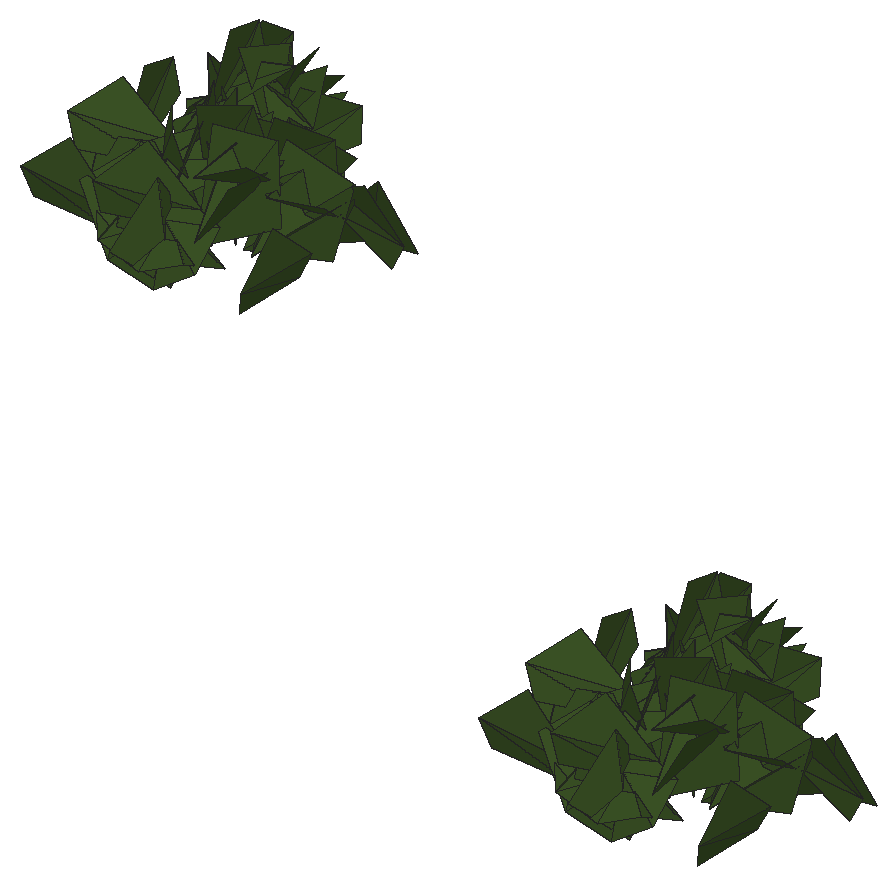
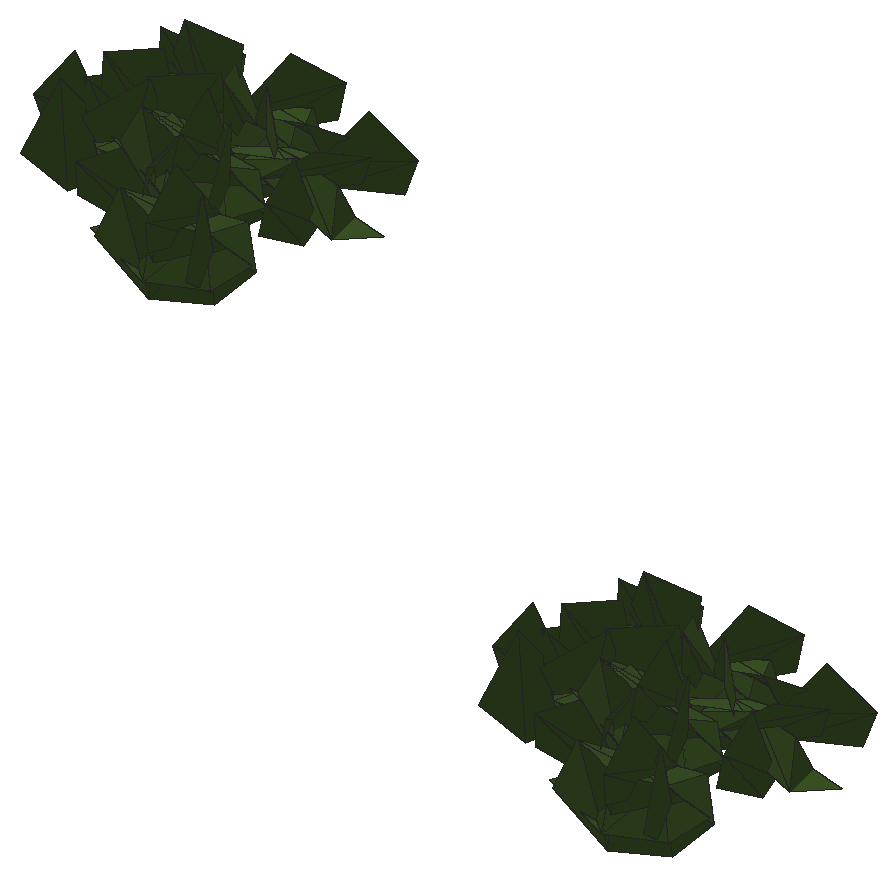
# SketchUp Ruby script. Lengths in inches.
U = 1.inch
M = Sketchup.active_model
def pt(a) = Geom::Point3d.new(a.map { |v| v * U })
def face(e, loops, mat)
  f = e.add_face(loops[0].map { |a| pt(a) })
  loops[1..].each { |l| e.add_face(l.map { |a| pt(a) }).erase! }
  f.material = f.back_material = mat if mat
  f
end
# faces: each face lists its corners as indices into pts; further lists are holes
def faces(e, pts, list, mat = nil) = list.each { |f| face(e, (f[0].is_a?(Array) ? f : [f]).map { |l| l.map { |i| pts[i] } }, mat) }
# xy, xz, yz: faces in a plane at the given z, y or x. An outline is a flat list of corners, or four numbers for a rectangle; further outlines are holes
def ring(l) = l.size == 4 ? [[l[0], l[1]], [l[2], l[1]], [l[2], l[3]], [l[0], l[3]]] : l.each_slice(2).to_a
def flat(e, list, mat, &to3) = list.each { |f| face(e, (f[0].is_a?(Array) ? f : [f]).map { |l| ring(l).map { |u, v| to3.(u, v) } }, mat) }
def xy(e, z, list, mat = nil) = flat(e, list, mat) { |x, y| [x, y, z] }
def xz(e, y, list, mat = nil) = flat(e, list, mat) { |x, z| [x, y, z] }
def yz(e, x, list, mat = nil) = flat(e, list, mat) { |y, z| [x, y, z] }
def lines(e, pts, list) = list.each { |a, b| e.add_line(pt(pts[a]), pt(pts[b])) }
# prism: a flat outline (further loops are holes) pulled along v
def prism(e, loops, v, mat = nil)
  f = face(e, loops, mat); d = Geom::Vector3d.new(v.map { |x| x * U })
  f.pushpull(f.normal.samedirection?(d) ? d.length : -d.length)
end
def box(e, o, s, mat = nil) = prism(e, [[o, [o[0] + s[0], o[1], o[2]], [o[0] + s[0], o[1] + s[1], o[2]], [o[0], o[1] + s[1], o[2]]]], [0, 0, s[2]], mat)
def at(x, y, z, deg = 0) = Geom::Transformation.translation(pt([x, y, z])) * Geom::Transformation.rotation(ORIGIN, Z_AXIS, deg.degrees)
def axes(o, x, y, z) = Geom::Transformation.new([*x, 0, *y, 0, *z, 0, *pt(o).to_a, 1])
def part(name) = M.definitions.add(name)
# library, detail: a bought-in or finely detailed component or shape, given as its bounding box
def library(name, o, s) = part(name).tap { |d| box(d.entities, o, s) }
def detail(e, o, s) = box(e.add_group.entities, o, s)
def put(e, d, t, mat = nil) = e.add_instance(d, t).tap { |i| i.material = mat if mat }
def group(e, t, mat = nil) = e.add_group.tap { |g| g.transformation = t; g.material = mat if mat }.entities
root = M.entities
M.materials.add("AM113_062_Tilia").color = [58, 81, 37]
p = [[1505.11,269.32,879.56],[1479.46,218.66,800.37],[1525.74,267.35,750.21],[1495.65,353.01,772.9],[344.49,918.09,879.56],[318.83,867.43,800.37],
  [365.11,916.125,750.21],[335.03,1001.78,772.9],[1444.78,257.76,760.62],[1516.15,249.39,752.03],[1512.28,272.93,827.79],[1563.2,262.4375,781.5],
  [284.15,906.53,760.62],[355.52,898.16,752.03],[351.66,921.7,827.79],[402.58,911.21,781.5],[1469.94,338.33,894.66],[1416.86,370.14,789.43],
  [1504.72,364.1,753.02],[309.3125,987.1,894.66],[256.24,1018.91,789.43],[344.09,1012.88,753.02],[1461.97,351.04,837.04],[1403.56,330.78,827.9],
  [1440.77,321.16,753.15],[1558.1,408.4,788.02],[301.35,999.8125,837.04],[242.93,979.56,827.9],[280.14,969.9375,753.15],[397.47,1057.18,788.02],
  [1384.37,557.68,884.94],[1368.75,544.08,755.59],[1451.59,506.93,778.28],[1365.28,611.16,805.75],[223.74,1206.46,884.94],[208.12,1192.85,755.59],
  [290.96,1155.71,778.28],[204.66,1259.9375,805.75],[1362.32,563.4,757.41],[1339.39,520.28,786.88],[1382.05,550,833.17],[1417.52,609.4,766],
  [201.69,1212.17,757.41],[178.76,1169.06,786.88],[221.43,1198.77,833.17],[256.89,1258.18,766],[1495.8,362.42,894.91],[1528.69,376.13,757.66],
  [1472.84,447.97,903.28],[1472.14,451.88,794.27],[335.17,1011.2,894.91],[368.07,1024.91,757.66],[312.22,1096.75,903.28],[311.52,1100.65,794.27],
  [1422.23,330.12,860.63],[1387.5,281.1,830.54],[1455.6,274.96,844.76],[261.61,978.89,860.63],[226.875,929.875,830.54],[294.97,923.73,844.76],
  [1685.92,428.47,868.25],[1643,469.68,760.75],[1601.23,388.02,775.93],[1718.77,458.36,776.85],[525.29,1077.24,868.25],[482.38,1118.45,760.75],
  [440.6,1036.8,775.93],[558.14,1107.14,776.85],[1558.49,353.8,770.9],[1643.65,403.42,764.22],[1669.83,408.41,867.79],[397.86,1002.58,770.9],
  [483.02,1052.19,764.22],[509.21,1057.1875,867.79],[1651.39,231.9,800.74],[1637.08,248.37,765.32],[1643.84,342.85,771.39],[490.77,880.68,800.74],
  [476.45,897.14,765.32],[483.21,991.625,771.39],[1510.12,285.74,822.95],[1557.17,250.19,797.3],[1562.42,315.02,765.59],[1425.7,366.6875,800.79],
  [349.49,934.51,822.95],[396.55,898.97,797.3],[401.8,963.8,765.59],[265.08,1015.46,800.79],[1422.54,589.72,850.14],[1485.52,575.95,866.01],
  [1473.88,634.88,835.92],[261.92,1238.49,850.14],[324.9,1224.72,866.01],[313.25,1283.66,835.92],[1353.5625,328.99,768.02],[1421.73,326.25,798.38],
  [1398.51,372.99,844.8],[1309.58,425.48,797.16],[1282.33,367.79,785.46],[1341.2,374.58,831.69],[192.9375,977.77,768.02],[261.1,975.03,798.38],
  [237.88,1021.76,844.8],[148.95,1074.26,797.16],[121.7,1016.57,785.46],[180.57,1023.35,831.69],[1565.52,422.83,908.3],[1570.57,466.93,789.28],
  [1547.93,378.67,768.94],[404.89,1071.6,908.3],[409.95,1115.71,789.28],[387.3,1027.45,768.94],[1585.97,394.56,901.01],[425.35,1043.33,901.01],
  [1413.57,298.3,770.99],[1430.23,294.69,796.45],[1312.58,269.91,826.9],[1320.73,282.97,786.25],[1392.83,542.75,828.34],[1334.66,533.09,802.68],
  [1378.07,484.65,770.97],[1509.66,548.26,806.17],[252.95,947.08,770.99],[269.6,943.47,796.45],[151.95,918.68,826.9],[160.1,931.75,786.25],
  [232.21,1191.52,828.34],[174.03,1181.86,802.68],[217.44,1133.42,770.97],[349.04,1197.03,806.17],[1487.9,508.69,771.26],[1468.25,501.02,791.03],
  [1561.72,556.84,863.53],[1564.38,550.76,819.11],[327.27,1157.47,771.26],[307.62,1149.79,791.03],[401.1,1205.62,863.53],[403.76,1199.53,819.11],
  [1653.78,354.39,798.69],[493.15,1003.17,798.69],[1350.65,421.7,773.0625],[1347.38,400.18,791.58],[1336.71,506.75,868.36],[1345.75,507.56,824.65],
  [190.03,1070.48,773.0625],[186.75,1048.96,791.58],[176.08,1155.53,868.36],[185.125,1156.34,824.65],[1501.6,378.68,917.83],[1544.36,423.41,812.6],
  [1519.05,339.0625,776.1875],[340.97,1027.45,917.83],[383.74,1072.1875,812.6],[358.43,987.84,776.1875],[1515.76,383.64,860.21],[1491.3125,410.92,776.32],
  [1550.46,277.21,811.19],[1508.92,445.09,851.07],[355.13,1032.41,860.21],[330.6875,1059.7,776.32],[389.83,925.99,811.19],[348.29,1093.86,851.07],
  [1437.12,249.91,786.11],[1509.2,232.2,779.4],[276.49,898.6875,786.11],[348.57,880.97,779.4],[1562.21,426.5625,847.86],[1513.07,446.8,780.26],
  [1594.53,322.58,788.5],[1545.51,486.28,841.09],[401.58,1075.34,847.86],[352.44,1095.58,780.26],[433.9,971.36,788.5],[384.88,1135.06,841.09],
  [1519.38,348.13,918.08],[1525.49,313.02,780.83],[1607.89,351.61,926.45],[1611.86,351.43,817.4375],[358.76,996.91,918.08],[364.86,961.8,780.83],
  [447.26,1000.38,926.45],[451.23,1000.2,817.4375],[1561.01,307.91,820.32],[400.38,956.69,820.32],[1743.47,403,818.28],[1723.06,407.125,781.875],
  [1632.79,427.18,809.1],[582.85,1051.77,818.28],[562.43,1055.9,781.875],[472.17,1075.95,809.1],[1354.63,580.28,784.78],[1417.1,620.36,791.49],
  [194.01,1229.05,784.78],[256.47,1269.13,791.49],[1432.96,463.53,862.68],[1378.53,452.98,826.2],[1430.25,418.54,785.93],[1548.78,487.1,860.66],
  [272.33,1112.3,862.68],[217.91,1101.76,826.2],[269.62,1067.32,785.93],[388.16,1135.88,860.66],[1387.74,308.3,825.5625],[1456.53,303.2,834.19],
  [227.11,957.08,825.5625],[295.9,951.98,834.19],[1373.89,490.57,825.7],[213.26,1139.35,825.7],[1504.99,386.93,850.82],[1457.88,435.22,860.24],
  [1539.46,446.22,863.7],[344.37,1035.7,850.82],[297.25,1084,860.24],[378.83,1094.99,863.7],[1595.99,380.64,850.07],[1652.01,340.6,839.9375],
  [1647.35,422.57,831.44],[435.36,1029.41,850.07],[491.38,989.38,839.9375],[486.73,1071.35,831.44],[1625.83,466.75,859.6],[465.21,1115.53,859.6],
  [1417.88,402.8,880.25],[257.25,1051.58,880.25],[1418.98,464.77,920.71],[1413.49,477.46,789.83],[1499.13,446.82,811.375],[1397.37,530.43,860],
  [258.35,1113.54,920.71],[252.86,1126.23,789.83],[338.5,1095.6,811.375],[236.75,1179.2,860],[1509.96,513.43,887.34],[349.33,1162.2,887.34],
  [1442.39,569.6,839.57],[1493.45,615.98,830.94],[281.77,1218.375,839.57],[332.82,1264.76,830.94],[1350.2,440.18,890.34],[189.57,1088.95,890.34],
  [1369.71,285.49,875.14],[209.08,934.27,875.14],[1404.27,494.76,797.14],[1386.01,444.67,807.44],[1420.98,468.16,868.16],[1451.6,543.28,829.08],
  [243.64,1143.54,797.14],[225.38,1093.45,807.44],[260.36,1116.94,868.16],[290.98,1192.06,829.08],[1448.34,406.71,840.37],[287.71,1055.48,840.37],
  [1458.1,353.11,836.26],[297.48,1001.88,836.26],[1654.98,283.26,861.98],[494.35,932.04,861.98],[1641.14,426.9,803.98],[1587.47,475.04,799.73],
  [1566.1875,436.48,858.54],[1536.8,483.98,820.48],[480.51,1075.68,803.98],[426.84,1123.81,799.73],[405.5625,1085.26,858.54],[376.17,1132.76,820.48],
  [1452.61,350.8,849.62],[1404.99,328.4375,804.51],[1453.57,303.7,801.14],[1550.84,398.52,862.69],[291.98,999.58,849.62],[244.36,977.21,804.51],
  [292.9375,952.48,801.14],[390.21,1047.29,862.69],[1516.07,306.08,803.74],[1530.72,314.36,829.44],[1438.53,238.91,866.41],[1441.8125,249.07,823.32],
  [355.45,954.85,803.74],[370.1,963.13,829.44],[277.9,887.6875,866.41],[281.18,897.85,823.32],[1522.33,454.83,826.1],[1485.1,544.58,803.8],
  [1452.22,568.22,899.62],[361.7,1103.6,826.1],[324.48,1193.36,803.8],[291.59,1217,899.62],[1606.37,334.47,861.7],[1665.35,360.27,857.73],
  [1609.52,399.375,873.5625],[445.74,983.24,861.7],[504.72,1009.04,857.73],[448.89,1048.15,873.5625],[1408.25,382.2,807.54],[247.625,1030.98,807.54],
  [1468.59,347.9,804.99],[1476.13,323.85,813.625],[1474.53,406.84,929.89],[1466.92,417.58,887.95],[307.96,996.67,804.99],[315.5,972.625,813.625],
  [313.91,1055.62,929.89],[306.29,1066.36,887.95],[1316.74,348.23,862.76],[1332.6,342.68,823.04],[1411.1,394.51,807.43],[1418.08,412.34,830.27],
  [1421.9,412.07,839.76],[156.11,997.01,862.76],[171.97,991.46,823.04],[250.47,1043.28,807.43],[257.45,1061.11,830.27],[261.27,1060.85,839.76],
  [1452.02,436.32,832.12],[291.4,1085.1,832.12],[1624.69,427.32,841.08],[1403.49,524.43,809.125],[1399.41,508.1,834.82],[1408.15,626.91,871.79],
  [1413.26,617.54,828.7],[464.0625,1076.09,841.08],[242.86,1173.2,809.125],[238.78,1156.88,834.82],[247.52,1275.6875,871.79],[252.63,1266.31,828.7],
  [1541.25,333.75,873.99],[1598.77,369.02,883.4],[1591.45,287.03,886.87],[380.625,982.52,873.99],[438.14,1017.8,883.4],[430.83,935.8,886.87],
  [1575.99,415.2,903.42],[415.37,1063.97,903.42],[1506.07,345.47,914.42],[345.44,994.25,914.42],[1696.3,391.8125,883.47],[535.67,1040.59,883.47],
  [1549.97,418.79,820.17],[1529.32,414.35,839.91],[1638.67,412.5,911.18],[1637.79,416.86,866.3],[389.34,1067.57,820.17],[368.69,1063.125,839.91],
  [478.04,1061.28,911.18],[477.16,1065.64,866.3],[1508.93,438.33,834.43],[348.3,1087.1,834.43],[1517.6,392.82,872.79],[1471.45,402.3,824.31],
  [1542.42,286.48,885.86],[1506.32,444.21,827.68],[356.97,1041.6,872.79],[310.83,1051.08,824.31],[381.79,935.25,885.86],[345.69,1092.98,827.68],
  [1448.78,482.53,929.4],[288.16,1131.31,929.4],[1392.58,504.16,827.92],[231.96,1152.9375,827.92],[1558.03,429.14,830.7],[397.4,1077.92,830.7],
  [1407.17,382.28,843.86],[1448.05,548.27,857.14],[246.55,1031.05,843.86],[287.42,1197.05,857.14],[1511.24,377.88,828.15],[1486.12,375.84,836.79],
  [1567.41,359.05,953.05],[1579.56,364.1,911.12],[350.61,1026.66,828.15],[325.49,1024.62,836.79],[406.78,1007.83,953.05],[418.9375,1012.88,911.12],
  [1454.19,507.19,903.82],[1517.32,498,923.76],[1499.24,559.3,913.04],[293.57,1155.97,903.82],[356.69,1146.78,923.76],[338.62,1208.08,913.04],
  [1477.625,286.375,909.65],[317,935.15,909.65],[1344.25,409.57,888.11],[183.625,1058.34,888.11],[1601.13,374.49,855.29],[440.51,1023.27,855.29],
  [1597.59,477.85,833.46],[436.96,1126.63,833.46],[1487.08,391.2,880.42],[1520.22,451.73,887.98],[326.45,1039.98,880.42],[359.59,1100.51,887.98],
  [1415.66,565.88,915.03],[255.04,1214.65,915.03],[1500.58,341.87,937.59],[339.96,990.64,937.59],[1447.28,451.36,839.68],[1444,429.84,858.2],
  [1433.33,536.41,934.97],[1442.375,537.22,891.27],[286.65,1100.14,839.68],[283.375,1078.62,858.2],[272.71,1185.19,934.97],[281.75,1186,891.27],
  [1574.7,387.16,928.06],[414.08,1035.9375,928.06],[1558.34,430.18,867.03],[397.72,1078.95,867.03],[1601.09,304.58,911.14],[1549.38,350.28,903.59],
  [440.46,953.35,911.14],[388.75,999.05,903.59],[1477.31,492.55,889.87],[1521.5625,544.6,904.81],[316.68,1141.32,889.87],[360.9375,1193.38,904.81],
  [1446.82,469.84,956.96],[286.19,1118.61,956.96]]
faces(root,p,[[0,1,2],[0,2,3],[4,5,6],[4,6,7],[8,9,10],[9,11,10],[12,13,14],[13,15,14],
  [16,17,18],[19,20,21],[22,23,24],[22,24,25],[26,27,28],[26,28,29],[30,31,32],[30,33,31],
  [34,35,36],[34,37,35],[38,39,40],[41,38,40],[42,43,44],[45,42,44],[46,47,48],[47,49,48],
  [50,51,52],[51,53,52],[54,55,8],[8,56,54],[10,56,8],[57,58,12],[12,59,57],[14,59,12],
  [60,61,62],[60,63,61],[64,65,66],[64,67,65],[68,69,70],[71,72,73],[74,75,76],[77,78,79],
  [80,81,82],[80,82,83],[84,85,86],[84,86,87],[40,88,41],[89,90,41],[41,88,89],[44,91,45],
  [92,93,45],[45,91,92],[94,95,96],[97,98,94],[94,99,97],[96,99,94],[100,101,102],[103,104,100],
  [100,105,103],[102,105,100],[106,107,108],[109,110,111],[112,68,70],[113,71,73],[114,115,116],[116,117,114],
  [118,119,120],[118,120,121],[122,123,124],[124,125,122],[126,127,128],[126,128,129],[130,131,132],[132,133,130],
  [134,135,136],[136,137,134],[76,138,74],[79,139,77],[140,141,142],[142,143,140],[144,145,146],[146,147,144],
  [148,149,150],[151,152,153],[154,155,156],[154,157,155],[158,159,160],[158,161,159],[162,163,80],[163,81,80],
  [164,165,84],[165,85,84],[166,167,168],[166,169,167],[170,171,172],[170,173,171],[174,175,176],[175,177,176],
  [178,179,180],[179,181,180],[10,11,182],[14,15,183],[184,185,186],[187,188,189],[190,119,118],[191,190,118],
  [192,127,126],[193,192,126],[194,195,196],[194,196,197],[198,199,200],[198,200,201],[83,202,162],[162,203,83],
  [80,203,162],[87,204,164],[164,205,87],[84,205,164],[40,39,206],[44,43,207],[25,208,22],[209,208,25],
  [25,210,209],[29,211,26],[212,211,29],[29,213,212],[168,214,166],[168,215,216],[216,214,168],[172,217,170],
  [172,218,219],[219,217,172],[106,220,107],[109,221,110],[16,222,17],[19,223,20],[224,225,226],[224,227,225],
  [228,229,230],[228,231,229],[131,232,132],[135,233,136],[118,234,191],[121,235,191],[191,234,121],[126,236,193],
  [129,237,193],[193,236,129],[141,238,142],[145,239,146],[115,240,116],[123,241,124],[242,243,244],[245,242,244],
  [246,247,248],[249,246,248],[96,250,97],[97,99,96],[102,251,103],[103,105,102],[95,252,96],[101,253,102],
  [138,254,74],[139,255,77],[256,257,258],[257,259,258],[260,261,262],[261,263,262],[83,203,80],[87,205,84],
  [264,265,266],[264,266,267],[268,269,270],[268,270,271],[272,273,274],[274,275,272],[276,277,278],[278,279,276],
  [280,281,282],[283,284,285],[286,287,256],[256,288,286],[258,288,256],[289,290,260],[260,291,289],[262,291,260],
  [292,265,264],[293,269,268],[294,295,296],[296,297,294],[298,299,300],[300,301,298],[121,234,118],[129,236,126],
  [302,303,304],[304,305,302],[244,243,306],[307,308,309],[309,310,307],[248,247,311],[312,292,264],[313,293,268],
  [186,314,184],[315,316,317],[317,318,315],[189,319,187],[320,321,322],[322,323,320],[156,324,154],[325,324,156],
  [156,326,325],[160,327,158],[328,327,160],[160,329,328],[148,330,149],[151,331,152],[295,332,296],[299,333,300],
  [314,334,184],[319,335,187],[336,337,338],[338,339,336],[340,341,342],[342,343,340],[10,182,54],[14,183,57],
  [258,259,344],[262,263,345],[346,347,348],[346,349,347],[350,351,352],[350,353,351],[40,206,89],[44,207,92],
  [354,280,282],[355,283,285],[356,195,194],[357,199,198],[358,349,346],[359,353,350],[54,56,10],[57,59,14],
  [360,23,22],[361,356,194],[362,27,26],[363,357,198],[364,365,366],[366,367,364],[368,369,370],[370,371,368],
  [244,372,245],[373,374,245],[245,372,373],[248,375,249],[376,377,249],[249,375,376],[273,378,274],[277,379,278],
  [305,380,302],[310,381,307],[382,358,346],[383,359,350],[166,214,216],[216,384,166],[170,217,219],[219,385,170],
  [264,386,312],[312,386,267],[267,387,312],[268,388,313],[313,388,271],[271,389,313],[89,88,40],[92,91,44],
  [384,169,166],[385,173,170],[258,344,286],[262,345,289],[316,390,317],[321,391,322],[96,252,250],[102,253,251],
  [365,392,366],[369,393,370],[209,360,22],[22,208,209],[212,362,26],[26,211,212],[394,395,396],[396,397,394],
  [398,399,400],[400,401,398],[244,306,373],[248,311,376],[337,402,338],[341,403,342],[267,386,264],[271,388,268],
  [404,157,154],[405,161,158],[348,406,382],[382,407,348],[346,407,382],[352,408,383],[383,409,352],[350,409,383],
  [194,410,361],[197,411,361],[361,410,197],[198,412,363],[201,413,363],[363,412,201],[395,414,396],[399,415,400],
  [286,288,258],[289,291,262],[154,324,325],[325,404,154],[158,327,328],[328,405,158],[197,410,194],[201,412,198],
  [373,372,244],[376,375,248],[348,407,346],[352,409,350]],"AM113_062_Tilia")
